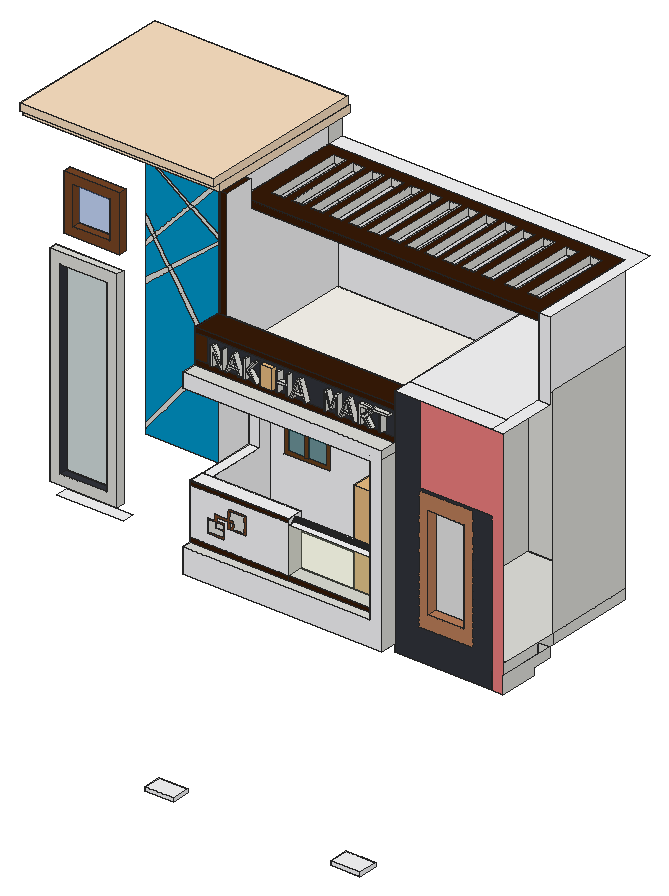
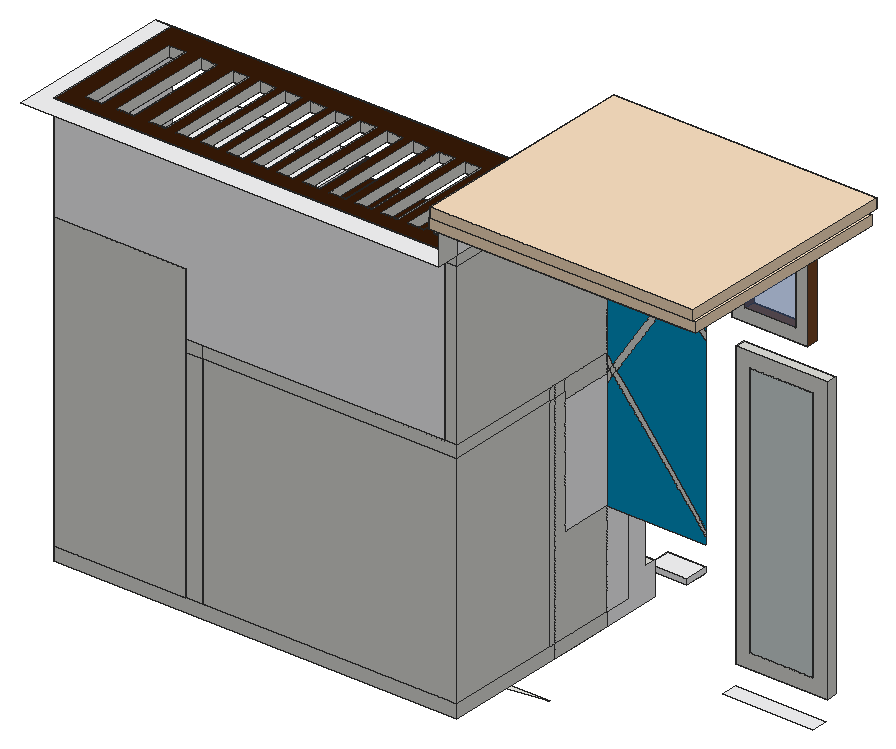
# SketchUp Ruby script. Lengths in inches.
U = 1.inch
M = Sketchup.active_model
def pt(a) = Geom::Point3d.new(a.map { |v| v * U })
def face(e, loops, mat)
  f = e.add_face(loops[0].map { |a| pt(a) })
  loops[1..].each { |l| e.add_face(l.map { |a| pt(a) }).erase! }
  f.material = f.back_material = mat if mat
  f
end
# faces: each face lists its corners as indices into pts; further lists are holes
def faces(e, pts, list, mat = nil) = list.each { |f| face(e, (f[0].is_a?(Array) ? f : [f]).map { |l| l.map { |i| pts[i] } }, mat) }
# xy, xz, yz: faces in a plane at the given z, y or x. An outline is a flat list of corners, or four numbers for a rectangle; further outlines are holes
def ring(l) = l.size == 4 ? [[l[0], l[1]], [l[2], l[1]], [l[2], l[3]], [l[0], l[3]]] : l.each_slice(2).to_a
def flat(e, list, mat, &to3) = list.each { |f| face(e, (f[0].is_a?(Array) ? f : [f]).map { |l| ring(l).map { |u, v| to3.(u, v) } }, mat) }
def xy(e, z, list, mat = nil) = flat(e, list, mat) { |x, y| [x, y, z] }
def xz(e, y, list, mat = nil) = flat(e, list, mat) { |x, z| [x, y, z] }
def yz(e, x, list, mat = nil) = flat(e, list, mat) { |y, z| [x, y, z] }
def lines(e, pts, list) = list.each { |a, b| e.add_line(pt(pts[a]), pt(pts[b])) }
# prism: a flat outline (further loops are holes) pulled along v
def prism(e, loops, v, mat = nil)
  f = face(e, loops, mat); d = Geom::Vector3d.new(v.map { |x| x * U })
  f.pushpull(f.normal.samedirection?(d) ? d.length : -d.length)
end
def box(e, o, s, mat = nil) = prism(e, [[o, [o[0] + s[0], o[1], o[2]], [o[0] + s[0], o[1] + s[1], o[2]], [o[0], o[1] + s[1], o[2]]]], [0, 0, s[2]], mat)
def at(x, y, z, deg = 0) = Geom::Transformation.translation(pt([x, y, z])) * Geom::Transformation.rotation(ORIGIN, Z_AXIS, deg.degrees)
def axes(o, x, y, z) = Geom::Transformation.new([*x, 0, *y, 0, *z, 0, *pt(o).to_a, 1])
def part(name) = M.definitions.add(name)
# library, detail: a bought-in or finely detailed component or shape, given as its bounding box
def library(name, o, s) = part(name).tap { |d| box(d.entities, o, s) }
def detail(e, o, s) = box(e.add_group.entities, o, s)
def put(e, d, t, mat = nil) = e.add_instance(d, t).tap { |i| i.material = mat if mat }
def group(e, t, mat = nil) = e.add_group.tap { |g| g.transformation = t; g.material = mat if mat }.entities
root = M.entities
M.materials.add("[0012_Bisque]").color = [255, 228, 196]
M.materials.add("[0013_LightCoral]1").color = [240, 128, 128]
M.materials.add("[0043_SaddleBrown]").color = [56, 27, 7]
M.materials.add("[0043_SaddleBrown]1").color = [79, 39, 10]
M.materials.add("[0097_DeepSkyBlue]").color = [0, 152, 204]
M.materials.add("[Asphalt New]").color = [84, 75, 77]
M.materials.add("[Blinds Vertical Pattern]").color = [250, 250, 252]
M.materials.add("[Color A08]").color = [66, 0, 0]
M.materials.add("[Formica Laminate Dark]").color = [50, 53, 60]
M.materials.add("[Formica Speckled Grey]").color = [94, 105, 111]
M.materials.add("[Sketchy Crosshatch Wavy]").color = [233, 233, 233]
M.materials.add("[Terrazzo Tile Light]").color = [255, 252, 244]
M.materials.add("[Translucent Glass Blue]").color = [78, 117, 186]
M.materials["[Translucent Glass Blue]"].alpha = 0.5
M.materials.add("[Translucent Glass Safety]").color = [227, 244, 187]
M.materials["[Translucent Glass Safety]"].alpha = 0.12
M.materials.add("[Translucent Glass Tinted]").color = [3, 87, 104]
M.materials["[Translucent Glass Tinted]"].alpha = 0.48
M.materials.add("[Wallpaper Dog Bone]").color = [213, 224, 224]
M.materials.add("[Wood Floor Parquet]").color = [104, 64, 28]
M.materials.add("[Wood Veneer 01]").color = [120, 70, 37]
M.materials.add("[Wood Veneer 02]").color = [190, 128, 91]
c1 = library("chau cay",[-24.34,-109.24,0],[56.46,62.58,79.69])
c2 = part("NAKSHA MART")
prism(c2.entities,[[[2.21,0.46,0],[2.21,19.72,0],[5.01,19.72,0],[13.81,5.77,0],[13.84,5.77,0],[13.84,19.72,0],[16.25,19.72,0],[16.25,0.46,0],[13.53,0.46,0],[4.67,14.54,0],[4.625,14.54,0],[4.625,0.46,0]]],[0,0,12])
prism(c2.entities,[[[18.64,0.46,0],[26.21,19.66,0],[29.16,19.66,0],[36.73,0.46,0],[33.61,0.46,0],[31.8,5.27,0],[23.03,5.27,0],[21.18,0.46,0]],[[23.91,7.48,0],[30.92,7.48,0],[27.4,16.65,0]]],[0,0,12])
prism(c2.entities,[[[76.07,0.46,0],[76.07,19.66,0],[79.02,19.66,0],[79.02,11.27,0],[87.14,11.27,0],[87.14,19.66,0],[90.09,19.66,0],[90.09,0.46,0],[87.14,0.46,0],[87.14,9.05,0],[79.02,9.05,0],[79.02,0.46,0]]],[0,0,12])
prism(c2.entities,[[[92.5,0.46,0],[100.07,19.66,0],[103.02,19.66,0],[110.59,0.46,0],[107.47,0.46,0],[105.66,5.27,0],[96.88,5.27,0],[95.04,0.46,0]],[[97.76,7.48,0],[104.77,7.48,0],[101.25,16.65,0]]],[0,0,12])
prism(c2.entities,[[[130.65,0.46,0],[130.65,19.66,0],[134.2,19.66,0],[138.42,7.84,0],[138.45,7.84,0],[142.59,19.66,0],[146.29,19.66,0],[146.29,0.46,0],[143.88,0.46,0],[143.88,16.9375,0],[143.85,16.9375,0],[139.53,4.52,0],[137.04,4.52,0],[132.73,16.59,0],[132.7,16.59,0],[132.7,0.46,0]]],[0,0,12])
prism(c2.entities,[[[147.89,0.46,0],[155.46,19.66,0],[158.41,19.66,0],[165.98,0.46,0],[162.86,0.46,0],[161.05,5.27,0],[152.27,5.27,0],[150.43,0.46,0]],[[153.16,7.48,0],[160.16,7.48,0],[156.64,16.65,0]]],[0,0,12])
prism(c2.entities,[[[168.93,0.46,0],[168.93,19.66,0],[174.3,19.66,0],[177.14,19.52,0],[178.95,19.11,0],[180.17,18.42,0],[181.04,17.51,0],[181.5625,16.39,0],[181.74,15.04,0],[181.49,13.2,0],[180.77,11.69,0],[179.48,10.4,0],[177.54,9.2,0],[184.17,0.46,0],[180.6,0.46,0],[174.54,8.45,0],[171.875,8.45,0],[171.875,0.46,0]],[[171.875,10.67,0],[173.43,10.67,0],[175.5625,10.93,0],[177.2,11.72,0],[177.8125,12.29,0],[178.25,12.95,0],[178.51,13.71,0],[178.59,14.55,0],[178.33,15.95,0],[178,16.46,0],[177.55,16.83,0],[176.06,17.29,0],[173.6875,17.45,0],[171.875,17.45,0]]],[0,0,12])
prism(c2.entities,[[[192.39,0.46,0],[192.39,17.45,0],[185.01,17.45,0],[185.01,19.66,0],[202.73,19.66,0],[202.73,17.45,0],[195.34,17.45,0],[195.34,0.46,0]]],[0,0,12])
xy(c2.entities,0,[[39.47,0.46,39.47,19.66,42.42,19.66,42.42,10.25,50.46,19.66,53.43,19.66,45.68,10.61,54.91,0.46,51.37,0.46,42.42,10.25,42.42,0.46]])
xy(c2.entities,12,[[39.47,0.46,42.42,0.46,42.42,10.25,51.37,0.46,54.91,0.46,45.68,10.61,53.43,19.66,50.46,19.66,42.42,10.25,42.42,19.66,39.47,19.66]])
xz(c2.entities,0.46,[[39.47,0,42.42,12],[51.37,0,54.91,12]])
xz(c2.entities,19.66,[[39.47,0,42.42,12],[50.46,0,53.43,12]])
yz(c2.entities,39.47,[[0.46,0,19.66,12]])
yz(c2.entities,42.42,[[0.46,0,10.25,12],[10.25,0,19.66,12]])
p = [[42.42,10.25,0],[51.37,0.46,0],[51.37,0.46,12],[42.42,10.25,12],[54.91,0.46,0],[45.68,10.61,0],
  [45.68,10.61,12],[54.91,0.46,12],[50.46,19.66,0],[50.46,19.66,12],[53.43,19.66,0],[53.43,19.66,12]]
faces(c2.entities,p,[[0,1,2,3],[4,5,6,7],[8,0,3,9],[5,10,11,6]])
detail(c2.entities,[57.85,0,0],[14.25,20.125,12])
xy(root,66.6875,[[328.59,26.375,349.16,29.3125],[198.03,27.5,217.83,29.3125],[198.03,29.3125,199.85,39.87],[199.85,29.3125,216.33,39.87],[216.33,29.3125,217.83,39.87],
  [328.59,29.3125,330.16,39.87],[330.16,29.3125,347.47,39.87],[347.47,29.3125,349.16,39.87]])
xy(root,69.375,[[328.59,26.375,349.16,39.87],[198.03,27.5,217.83,39.87]],"[Blinds Vertical Pattern]")
xy(root,108.13,[[239.11,191.13,244.8,194.19],[247.86,191.13,253.55,194.19],[256.61,191.13,262.3,194.19],[265.86,191.13,271.55,194.19]],"[Formica Laminate Dark]")
xy(root,124.1875,[[271.54,153.45,339.34,194.19],[339.34,153.45,347.47,180.38]],"[Formica Laminate Dark]")
xy(root,125.11,[[19.23,173.82,65.86,182.32]],"[Blinds Vertical Pattern]")
xy(root,127.39,[[239.11,191.13,244.8,194.19],[247.86,191.13,253.55,194.19],[256.61,191.13,262.3,194.19],[265.86,191.13,271.55,194.19]])
xy(root,129,[[[132.29,142.51,271.54,194.19],[133.75,159.42,143.75,170.29]],[339.34,180.38,347.47,194.19],[132.29,194.19,339.34,207.2],[132.29,207.2,339.34,270.27]])
xy(root,135.61,[[18.61,168.38,65.8,173.82]])
xy(root,136,[[132.29,159.82,139.39,210.08],[271.54,166.83,339.34,270.27],[132.29,210.08,262.84,270.27]])
xy(root,136,[[139.39,159.82,262.84,210.08]],"[Terrazzo Tile Light]")
xy(root,143.06,[[26.07,168.38,58.34,173.82]],"[Formica Laminate Dark]")
xy(root,146.0625,[[132.29,142.51,262.84,148.875]])
xy(root,149.125,[[201.12,148.875,262.84,159.82]])
xy(root,155.77,[[294.84,153.45,320.31,160.63]],"[Wood Veneer 02]")
xy(root,180.75,[[201.12,148.875,262.84,159.82]],"[Blinds Vertical Pattern]")
xy(root,184.6875,[[132.29,148.875,201.12,159.82],[132.29,159.82,139.39,200.69]])
xy(root,184.75,[[132.29,148.875,201.12,159.82],[132.29,159.82,139.39,200.69]],"[Blinds Vertical Pattern]")
xy(root,221.125,[[294.84,153.45,320.31,160.63]],"[Wood Veneer 02]")
xy(root,245.625,[[132.29,142.51,132.29,200.69,139.39,200.69,139.39,210.08,262.84,210.08,262.84,142.51]],"[Terrazzo Tile Light]")
xy(root,249,[[262.84,167.76,271.54,210.08],[132.29,200.69,139.39,210.08],[132.29,210.08,262.84,270.27],[262.84,210.08,271.54,270.27]])
xy(root,255.1875,[[132.29,142.51,271.54,153.45],[132.29,153.45,271.54,173.82],[132.29,173.82,138.29,200.69],[132.29,200.69,138.29,207.2],[132.29,207.2,138.29,210.08],
  [132.29,210.08,138.29,270.27]])
xy(root,255.1875,[[138.29,173.82,271.54,270.27]],"[Terrazzo Tile Light]")
xy(root,274.4,[[26.07,168.38,58.34,173.82]],"[Formica Laminate Dark]")
xy(root,275.125,[[132.29,153.45,271.54,173.82]])
xy(root,278.625,[[132.29,153.45,271.54,173.82]],"[0043_SaddleBrown]")
xy(root,281.86,[[18.61,168.38,65.8,173.82]])
xy(root,287.6875,[[271.54,153.45,339.34,166.83],[339.34,153.45,347.47,194.64],[271.54,166.83,339.34,270.27]],"[Blinds Vertical Pattern]")
xy(root,294.76,[[28.5625,168.13,67.5625,173.82]],"[Wood Veneer 01]")
xy(root,301.09,[[34.89,168.13,61.24,173.82]],"[Wood Veneer 01]")
xy(root,327.44,[[34.89,168.13,61.24,173.82]],"[Wood Veneer 01]")
xy(root,333.76,[[28.5625,168.13,67.5625,173.82]],"[Wood Veneer 01]")
xy(root,337.4,[[132.29,194.64,138.29,270.27]])
xy(root,337.4,[[[138.29,194.64,339.34,270.27],[142.56,207.87,151.06,261.56],[156,207.87,164.5,261.56],[169.44,207.87,177.94,261.56],[182.87,207.87,191.37,261.56],[196.31,207.87,204.81,261.56],[209.75,207.87,218.25,261.56],[223.19,207.87,231.69,261.56],[236.12,207.87,244.62,261.56],[249.06,207.87,257.56,261.56],[262,207.87,270.5,261.56],[274.94,207.87,283.44,261.56],[321.5,207.87,330,261.56],[288.87,207.87,297.37,261.56],[305.25,207.87,313.75,261.56]]],"[0043_SaddleBrown]")
xy(root,342.375,[[[132.29,194.64,339.34,270.27],[142.56,207.87,151.06,261.56],[156,207.87,164.5,261.56],[169.44,207.87,177.94,261.56],[182.87,207.87,191.37,261.56],[196.31,207.87,204.81,261.56],[209.75,207.87,218.25,261.56],[223.19,207.87,231.69,261.56],[236.12,207.87,244.62,261.56],[249.06,207.87,257.56,261.56],[262,207.87,270.5,261.56],[274.94,207.87,283.44,261.56],[288.87,207.87,297.37,261.56],[305.25,207.87,313.75,261.56],[321.5,207.87,330,261.56]]],"[0043_SaddleBrown]")
xy(root,342.375,[[339.34,194.64,347.47,194.64,347.47,281.71,132.29,281.71,132.29,270.27,339.34,270.27]],"[Blinds Vertical Pattern]")
xy(root,355.27,[[132.29,173.82,138.29,194.64]],"[0043_SaddleBrown]")
xy(root,358.25,[[5.9375,173.82,132.29,281.71],[132.29,194.64,137.48,270.27],[132.29,270.27,137.48,281.71]])
xy(root,358.25,[[0,168.63,17.38,173.82],[17.38,168.63,137.48,173.82],[0,173.82,5.9375,281.71],[132.29,173.82,137.48,194.64]],"[0012_Bisque]")
xy(root,363.3125,[[1.4375,168.63,136.67,281.71]])
xy(root,363.3125,[[1.4375,163.88,136.67,168.63],[0,168.63,1.4375,281.71],[136.67,168.63,137.48,281.71]],"[0012_Bisque]")
xy(root,368.5,[[1.4375,163.88,136.67,281.71]],"[0012_Bisque]")
xz(root,26.375,[[328.59,66.6875,349.16,69.375]],"[Blinds Vertical Pattern]")
xz(root,27.5,[[198.03,66.6875,217.83,69.375]],"[Blinds Vertical Pattern]")
xz(root,39.87,[[198.03,66.6875,217.83,69.375],[328.59,66.6875,334.94,69.375],[334.94,66.6875,339.34,69.375],[339.34,66.6875,349.16,69.375]],"[Blinds Vertical Pattern]")
xz(root,142.51,[[132.29,129,271.54,129,271.54,255.1875,132.29,255.1875,132.29,245.625,262.84,245.625,262.84,146.0625,132.29,146.0625]],"[Blinds Vertical Pattern]")
xz(root,148.875,[[145.74,157.27,155.1,157.27,155.1,160.82,149.79,160.82,149.79,164.57,145.74,164.57],[151.1,161.72,155.1,164.57],[159.85,164.57,161.67,167.94],[163.04,164.57,170.04,164.57,170.04,174.88,159.85,174.88,159.85,169.63,163.04,169.63],[132.29,184.6875,201.12,184.75]])
xz(root,148.875,[[132.29,146.0625,201.12,149.125],[201.12,146.0625,262.84,149.125],[132.29,181.99,201.12,184.6875]],"[0043_SaddleBrown]")
xz(root,148.875,[[[132.29,149.125,201.12,181.99],[144.58,156.11,144.58,165.73,149.79,165.73,149.79,169.63,158.99,169.63,158.99,176.01,171.24,176.01,171.24,163.51,158.99,163.51,158.99,167.94,151.1,167.94,151.1,165.73,156.26,165.73,156.26,156.11]]],"[Blinds Vertical Pattern]")
xz(root,148.875,[[201.12,149.125,262.84,180.75]],"[Translucent Glass Safety]")
xz(root,148.875,[[[144.58,156.11,156.26,156.11,156.26,165.73,151.1,165.73,151.1,167.94,158.99,167.94,158.99,163.51,171.24,163.51,171.24,176.01,158.99,176.01,158.99,169.63,149.79,169.63,149.79,165.73,144.58,165.73],[163.04,164.57,163.04,169.63,159.85,169.63,159.85,174.88,170.04,174.88,170.04,164.57],[145.74,157.27,145.74,164.57,149.79,164.57,149.79,160.82,155.1,160.82,155.1,161.72,151.1,161.72,151.1,164.57,155.1,164.57,155.1,157.27],[159.85,164.57,161.67,167.94]]],"[Wood Veneer 01]")
xz(root,153.45,[[339.34,124.1875,347.47,124.1875,347.47,287.6875,289.09,287.6875,289.09,233.28,339.34,233.28]],"[0013_LightCoral]1")
xz(root,153.45,[[132.29,255.1875,271.54,258.83],[132.29,275.125,271.54,278.625]],"[0043_SaddleBrown]")
xz(root,153.45,[[132.29,258.83,140.34,275.125]],"[0043_SaddleBrown]1")
xz(root,153.45,[[271.54,124.1875,339.34,124.1875,339.34,233.28,289.09,233.28,289.09,231.5,326.23,231.5,326.23,145.9375,288.92,145.9375,288.92,231.5,289.09,231.5,289.09,287.6875,271.54,287.6875],[140.34,258.83,271.54,275.125]],"[Formica Laminate Dark]")
xz(root,153.45,[[[288.92,145.9375,326.23,231.5],[294.84,155.77,320.31,221.125]]],"[Wood Veneer 02]")
xz(root,159.82,[[132.29,136,139.39,184.6875],[132.29,184.6875,139.39,184.75],[139.39,184.6875,201.12,184.75]])
xz(root,159.82,[[139.39,136,139.39,184.6875,201.12,184.6875,201.12,149.125,262.84,149.125,262.84,136]],"[Blinds Vertical Pattern]")
xz(root,159.82,[[201.12,149.125,262.84,180.75]],"[Translucent Glass Safety]")
xz(root,160.63,[[294.84,155.77,320.31,221.125]],"[Sketchy Crosshatch Wavy]")
xz(root,163.88,[[1.4375,363.3125,136.67,368.5]],"[0012_Bisque]")
xz(root,168.13,[[[28.5625,294.76,67.5625,333.76],[34.89,301.09,61.24,327.44]]],"[Wood Veneer 01]")
xz(root,168.38,[[[18.61,135.61,65.8,281.86],[26.07,143.06,58.34,274.4]]])
xz(root,168.63,[[0,358.25,137.48,363.3125]],"[0012_Bisque]")
xz(root,173.82,[[[18.61,135.61,65.8,281.86],[26.07,143.06,58.34,274.4]],[81.27,188.4,128.85,246.23,127.14,248.81,81.27,191.96],[132.29,241.04,132.29,245.625,130.55,248.28,128.85,246.23],[132.29,245.625,132.29,250.41,130.55,248.28],[128.85,246.23,130.55,248.28,128.83,250.89,127.14,248.81],
  [130.55,248.28,132.29,250.41,132.29,255.1875,128.83,250.89],[127.14,248.81,128.83,250.89,100.1,294.61,97.95,292.84],[132.29,255.1875,138.29,275.125],[132.29,275.125,133.19,278.625],[133.19,275.125,138.29,278.625],
  [132.29,278.625,133.19,355.27],[81.27,279.07,97.95,292.84,96.41,295.17,81.27,283],[97.95,292.84,100.1,294.61,98.58,296.91,96.41,295.17],[100.1,294.61,132.29,321.1875,132.29,324.01,98.58,296.91],[[28.5625,294.76,67.5625,333.76],[34.89,301.09,61.24,327.44]],
  [96.41,295.17,98.58,296.91,89.2,311.1875,87.22,309.02],[81.27,302.53,87.22,309.02,85.9,311.01,81.27,305.99],[87.22,309.02,89.2,311.1875,87.9,313.17,85.9,311.01],[85.9,311.01,87.9,313.17,81.27,323.25,81.27,317.99],[89.2,311.1875,112.875,337.04,111.05,338.27,87.9,313.17],
  [132.29,324.01,132.29,327.53,114.8,339.14,112.875,337.04],[112.875,337.04,114.8,339.14,112.97,340.36,111.05,338.27],[111.05,338.27,112.97,340.36,86.01,358.25,81.27,358.25],[114.8,339.14,132.29,358.25,129.47,358.25,112.97,340.36]])
xz(root,173.82,[[133.19,278.625,138.29,355.27]],"[0043_SaddleBrown]")
xz(root,173.82,[[132.29,184.75,132.29,241.04,128.85,246.23,81.27,188.4,81.27,184.84],[81.27,191.96,127.14,248.81,97.95,292.84,81.27,279.07],[128.83,250.89,132.29,255.1875,132.29,321.1875,100.1,294.61],[81.27,283,96.41,295.17,87.22,309.02,81.27,302.53],[98.58,296.91,132.29,324.01,112.875,337.04,89.2,311.1875],
  [81.27,305.99,85.9,311.01,81.27,317.99],[87.9,313.17,111.05,338.27,81.27,358.25,81.27,323.25],[132.29,327.53,132.29,358.25,114.8,339.14],[112.97,340.36,129.47,358.25,86.01,358.25]],"[0097_DeepSkyBlue]")
xz(root,173.82,[[138.29,255.1875,271.54,275.125],[138.29,275.125,271.54,278.625]],"[Color A08]")
xz(root,173.82,[[34.89,301.09,61.24,327.44]],"[Translucent Glass Blue]")
xz(root,173.82,[[26.07,143.06,58.34,274.4]],"[Wallpaper Dog Bone]")
xz(root,180.38,[[339.34,124.1875,347.47,129]])
xz(root,191.13,[[239.11,108.13,244.8,127.39],[247.86,108.13,253.55,127.39],[256.61,108.13,262.3,127.39],[265.86,108.13,271.55,127.39]],"[Formica Laminate Dark]")
xz(root,194.19,[[239.11,108.13,244.8,127.39],[247.86,108.13,253.55,127.39],[256.61,108.13,262.3,127.39],[265.86,108.13,265.86,127.39,271.54,127.39,271.54,124.1875,271.55,124.1875,271.55,108.13],[271.54,124.1875,271.55,127.39],
  [271.55,124.1875,287,124.1875,287,129,271.54,129,271.54,127.39,271.55,127.39],[287,124.1875,339.34,129],[339.34,129,347.47,136]])
xz(root,194.64,[[132.29,337.4,138.29,342.375],[132.29,342.375,138.29,355.27]])
xz(root,194.64,[[138.29,337.4,339.34,342.375]],"[0043_SaddleBrown]")
xz(root,194.64,[[339.34,287.6875,347.47,342.375]],"[Blinds Vertical Pattern]")
xz(root,200.69,[[132.29,184.6875,139.39,184.75],[132.29,245.625,139.39,249]])
xz(root,200.69,[[132.29,184.75,139.39,245.625]],"[Blinds Vertical Pattern]")
xz(root,207.87,[[142.56,337.4,151.06,342.375],[156,337.4,164.5,342.375],[169.44,337.4,177.94,342.375],[182.87,337.4,191.37,342.375],[196.31,337.4,204.81,342.375],
  [209.75,337.4,218.25,342.375],[223.19,337.4,231.69,342.375],[236.12,337.4,244.62,342.375],[249.06,337.4,257.56,342.375],[262,337.4,270.5,342.375],
  [274.94,337.4,283.44,342.375],[288.87,337.4,297.37,342.375],[305.25,337.4,313.75,342.375],[321.5,337.4,330,342.375]])
xz(root,210.08,[[132.29,136,139.39,249],[139.39,245.625,262.84,249]])
xz(root,210.08,[[[139.39,136,262.84,245.625],[212.31,140.93,240.81,230.93],[149.18,180.3125,181.93,229.875]]],"[Blinds Vertical Pattern]")
xz(root,210.08,[[216.73,145.34,236.4,226.52],[152.18,183.31,163.88,226.875],[166.375,183.31,178.93,226.875]],"[Translucent Glass Tinted]")
xz(root,210.08,[[[212.31,140.93,240.81,230.93],[216.73,145.34,236.4,226.52]],[[149.18,180.3125,181.93,229.875],[152.18,183.31,178.93,226.875]],[163.88,183.31,166.375,226.875]],"[Wood Floor Parquet]")
xz(root,261.56,[[142.56,337.4,151.06,342.375],[156,337.4,164.5,342.375],[169.44,337.4,177.94,342.375],[182.87,337.4,191.37,342.375],[196.31,337.4,204.81,342.375],
  [209.75,337.4,218.25,342.375],[223.19,337.4,231.69,342.375],[236.12,337.4,244.62,342.375],[249.06,337.4,257.56,342.375],[262,337.4,270.5,342.375],
  [274.94,337.4,283.44,342.375],[288.87,337.4,297.37,342.375],[305.25,337.4,313.75,342.375],[321.5,337.4,330,342.375]])
xz(root,270.27,[[132.29,129,339.34,136],[132.29,136,262.84,249],[262.84,136,271.54,249],[271.54,136,339.34,287.6875],[132.29,249,262.84,255.1875],
  [262.84,249,271.54,255.1875],[132.29,255.1875,138.29,337.4],[132.29,337.4,339.34,342.375]])
xz(root,270.27,[[138.29,255.1875,271.54,255.1875,271.54,287.6875,339.34,287.6875,339.34,337.4,138.29,337.4]],"[Blinds Vertical Pattern]")
xz(root,281.71,[[0,358.25,137.48,363.3125],[1.4375,363.3125,136.67,368.5]],"[0012_Bisque]")
yz(root,0,[[168.63,358.25,281.71,363.3125]],"[0012_Bisque]")
yz(root,1.4375,[[163.88,363.3125,281.71,368.5]],"[0012_Bisque]")
yz(root,18.61,[[168.38,135.61,173.82,281.86]])
yz(root,26.07,[[168.38,143.06,173.82,274.4]],"[Formica Laminate Dark]")
yz(root,28.5625,[[168.13,294.76,173.82,333.76]],"[Wood Veneer 01]")
yz(root,34.89,[[168.13,301.09,173.82,327.44]],"[Wood Veneer 01]")
yz(root,58.34,[[168.38,143.06,173.82,274.4]],"[Formica Laminate Dark]")
yz(root,61.24,[[168.13,301.09,173.82,327.44]],"[Wood Veneer 01]")
yz(root,65.8,[[168.38,135.61,173.82,281.86]])
yz(root,67.5625,[[168.13,294.76,173.82,333.76]],"[Wood Veneer 01]")
yz(root,132.29,[[173.82,129,207.2,136],[207.2,129,270.27,136],[173.82,136,207.2,136,207.2,249,200.69,249,200.69,184.6875,173.82,184.6875],[207.2,136,210.08,249],[210.08,136,270.27,249],
  [148.875,184.6875,159.82,184.75],[159.82,184.6875,173.82,184.75],[173.82,184.6875,200.69,184.75],[142.51,245.625,173.82,255.1875],[173.82,245.625,200.69,255.1875],
  [200.69,249,207.2,255.1875],[207.2,249,210.08,255.1875],[210.08,249,270.27,255.1875],[173.82,255.1875,173.82,355.27,194.64,355.27,194.64,337.4,270.27,337.4,270.27,255.1875],[194.64,337.4,270.27,342.375],
  [270.27,342.375,281.71,358.25]])
yz(root,132.29,[[142.51,129,142.51,146.0625,148.875,146.0625,148.875,184.6875,159.82,184.6875,159.82,136,173.82,136,173.82,129],[159.82,136,173.82,184.6875],[173.82,184.75,200.69,245.625],[194.64,342.375,270.27,358.25],[173.82,355.27,194.64,358.25]],"[Blinds Vertical Pattern]")
yz(root,132.29,[[153.45,255.1875,173.82,275.125],[153.45,275.125,173.82,278.625]],"[Color A08]")
yz(root,136.67,[[163.88,363.3125,281.71,368.5]],"[0012_Bisque]")
yz(root,137.48,[[168.63,358.25,281.71,363.3125]],"[0012_Bisque]")
yz(root,138.29,[[173.82,255.1875,270.27,255.1875,270.27,337.4,194.64,337.4,194.64,355.27,173.82,355.27]],"[Blinds Vertical Pattern]")
yz(root,139.39,[[159.82,184.6875,200.69,184.75],[200.69,245.625,210.08,249]])
yz(root,139.39,[[159.82,136,210.08,136,210.08,245.625,200.69,245.625,200.69,184.6875,159.82,184.6875]],"[Blinds Vertical Pattern]")
yz(root,142.56,[[207.87,337.4,261.56,342.375]])
yz(root,151.06,[[207.87,337.4,261.56,342.375]])
yz(root,156,[[207.87,337.4,261.56,342.375]])
yz(root,164.5,[[207.87,337.4,261.56,342.375]])
yz(root,169.44,[[207.87,337.4,261.56,342.375]])
yz(root,177.94,[[207.87,337.4,261.56,342.375]])
yz(root,182.87,[[207.87,337.4,261.56,342.375]])
yz(root,191.37,[[207.87,337.4,261.56,342.375]])
yz(root,196.31,[[207.87,337.4,261.56,342.375]])
yz(root,198.03,[[27.5,66.6875,39.87,69.375]],"[Blinds Vertical Pattern]")
yz(root,201.12,[[148.875,149.125,159.82,180.75],[154.07,181.21,153.74,181.25,153.44,181.375,153.18,181.57,152.99,181.83,152.86,182.13,152.82,182.46,152.86,182.78,152.99,183.08,153.18,183.34,153.44,183.54,153.74,183.66,154.07,183.71,154.39,183.66,154.69,183.54,154.95,183.34,155.15,183.08,155.28,182.78,155.32,182.46,155.28,182.13,155.15,181.83,154.95,181.57,154.69,181.375,154.39,181.25],[148.875,184.6875,159.82,184.75]])
yz(root,201.12,[[[148.875,180.75,159.82,184.6875],[154.07,181.21,153.74,181.25,153.44,181.375,153.18,181.57,152.99,181.83,152.86,182.13,152.82,182.46,152.86,182.78,152.99,183.08,153.18,183.34,153.44,183.54,153.74,183.66,154.07,183.71,154.39,183.66,154.69,183.54,154.95,183.34,155.15,183.08,155.28,182.78,155.32,182.46,155.28,182.13,155.15,181.83,154.95,181.57,154.69,181.375,154.39,181.25]]],"[Blinds Vertical Pattern]")
yz(root,204.81,[[207.87,337.4,261.56,342.375]])
yz(root,209.75,[[207.87,337.4,261.56,342.375]])
yz(root,217.83,[[27.5,66.6875,39.87,69.375]],"[Blinds Vertical Pattern]")
yz(root,218.25,[[207.87,337.4,261.56,342.375]])
yz(root,223.19,[[207.87,337.4,261.56,342.375]])
yz(root,231.69,[[207.87,337.4,261.56,342.375]])
yz(root,236.12,[[207.87,337.4,261.56,342.375]])
yz(root,239.11,[[191.13,108.13,194.19,127.39]],"[Formica Laminate Dark]")
yz(root,244.62,[[207.87,337.4,261.56,342.375]])
yz(root,244.8,[[191.13,108.13,194.19,127.39]],"[Formica Laminate Dark]")
yz(root,247.86,[[191.13,108.13,194.19,127.39]],"[Formica Laminate Dark]")
yz(root,249.06,[[207.87,337.4,261.56,342.375]])
yz(root,253.55,[[191.13,108.13,194.19,127.39]],"[Formica Laminate Dark]")
yz(root,256.61,[[191.13,108.13,194.19,127.39]],"[Formica Laminate Dark]")
yz(root,257.56,[[207.87,337.4,261.56,342.375]])
yz(root,262,[[207.87,337.4,261.56,342.375]])
yz(root,262.3,[[191.13,108.13,194.19,127.39]],"[Formica Laminate Dark]")
yz(root,262.84,[[210.08,136,270.27,249],[148.875,149.125,159.82,180.75],[167.76,245.625,210.08,249]])
yz(root,262.84,[[159.82,136,159.82,146.0625,167.76,146.0625,167.76,245.625,210.08,245.625,210.08,136],[[142.51,146.0625,142.51,245.625,167.76,245.625,167.76,146.0625,159.82,146.0625,159.82,180.75,148.875,180.75,148.875,146.0625],[154.07,181.21,154.39,181.25,154.69,181.375,154.95,181.57,155.15,181.83,155.28,182.13,155.32,182.46,155.28,182.78,155.15,183.08,154.95,183.34,154.69,183.54,154.39,183.66,154.07,183.71,153.74,183.66,153.44,183.54,153.18,183.34,152.99,183.08,152.86,182.78,152.82,182.46,152.86,182.13,152.99,181.83,153.18,181.57,153.44,181.375,153.74,181.25]]],"[Blinds Vertical Pattern]")
yz(root,265.86,[[191.13,108.13,194.19,127.39]],"[Formica Laminate Dark]")
yz(root,270.5,[[207.87,337.4,261.56,342.375]])
yz(root,271.54,[[153.45,124.1875,194.19,129],[142.51,129,153.45,249],[166.83,136,270.27,136,270.27,249,167.76,249,167.76,255.1875,166.83,255.1875],[142.51,249,153.45,255.1875],[167.76,249,210.08,255.1875],
  [210.08,249,270.27,255.1875],[153.45,255.1875,166.83,275.125],[166.83,255.1875,167.76,275.125],[167.76,255.1875,173.82,275.125],[153.45,275.125,166.83,278.625],
  [166.83,275.125,167.76,278.625],[167.76,275.125,173.82,278.625]])
yz(root,271.54,[[153.45,278.625,166.83,287.6875]],"[Asphalt New]")
yz(root,271.54,[[173.82,255.1875,173.82,278.625,166.83,278.625,166.83,287.6875,210.08,287.6875,210.08,255.1875],[210.08,255.1875,270.27,287.6875]],"[Blinds Vertical Pattern]")
yz(root,271.55,[[191.13,108.13,194.19,127.39]],"[Formica Laminate Dark]")
yz(root,274.94,[[207.87,337.4,261.56,342.375]])
yz(root,283.44,[[207.87,337.4,261.56,342.375]])
yz(root,288.87,[[207.87,337.4,261.56,342.375]])
yz(root,294.84,[[153.45,155.77,160.63,221.125]],"[Wood Veneer 02]")
yz(root,297.37,[[207.87,337.4,261.56,342.375]])
yz(root,305.25,[[207.87,337.4,261.56,342.375]])
yz(root,313.75,[[207.87,337.4,261.56,342.375]])
yz(root,320.31,[[153.45,155.77,160.63,221.125]],"[Wood Veneer 02]")
yz(root,321.5,[[207.87,337.4,261.56,342.375]])
yz(root,328.59,[[26.375,66.6875,39.87,69.375]],"[Blinds Vertical Pattern]")
yz(root,330,[[207.87,337.4,261.56,342.375]])
yz(root,339.34,[[153.45,124.1875,180.38,124.1875,180.38,129,194.19,129,194.19,136,153.45,136],[180.38,124.1875,194.19,129],[194.19,129,207.2,136],[207.2,129,270.27,136],[207.2,136,270.27,287.6875],
  [194.64,337.4,270.27,342.375]])
yz(root,339.34,[[194.64,287.6875,270.27,337.4]],"[Blinds Vertical Pattern]")
yz(root,347.47,[[153.45,124.1875,180.38,124.1875,180.38,129,194.19,129,194.19,136,153.45,136]])
yz(root,349.16,[[26.375,66.6875,39.87,69.375]],"[Blinds Vertical Pattern]")
p = [[145.06,194.19,99.57],[158.57,207.2,106.65],[218.13,207.2,106.65],[197.47,194.19,99.57],[201.12,153.44,181.375],[201.12,153.74,181.25],
  [262.84,153.74,181.25],[262.84,153.44,181.375],[201.12,154.07,181.21],[262.84,154.07,181.21],[201.12,154.39,181.25],[262.84,154.39,181.25],
  [201.12,154.69,181.375],[262.84,154.69,181.375],[201.12,153.18,181.57],[262.84,153.18,181.57],[201.12,154.95,181.57],[262.84,154.95,181.57],
  [201.12,152.99,181.83],[262.84,152.99,181.83],[201.12,155.15,181.83],[262.84,155.15,181.83],[201.12,152.86,182.13],[262.84,152.86,182.13],
  [201.12,155.28,182.13],[262.84,155.28,182.13],[201.12,152.82,182.46],[262.84,152.82,182.46],[201.12,155.32,182.46],[262.84,155.32,182.46],
  [201.12,152.86,182.78],[262.84,152.86,182.78],[201.12,155.28,182.78],[262.84,155.28,182.78],[201.12,152.99,183.08],[262.84,152.99,183.08],
  [201.12,155.15,183.08],[262.84,155.15,183.08],[201.12,153.18,183.34],[262.84,153.18,183.34],[201.12,154.95,183.34],[262.84,154.95,183.34],
  [201.12,153.44,183.54],[262.84,153.44,183.54],[201.12,154.69,183.54],[262.84,154.69,183.54],[201.12,153.74,183.66],[262.84,153.74,183.66],
  [201.12,154.39,183.66],[262.84,154.39,183.66],[201.12,154.07,183.71],[262.84,154.07,183.71],[262.84,159.82,136],[262.84,153.45,136],
  [262.84,167.76,249],[262.84,142.51,249]]
faces(root,p,[[0,1,2,3]])
faces(root,p,[[4,5,6,7],[5,8,9,6],[8,10,11,9],[10,12,13,11],[14,4,7,15],[12,16,17,13],[18,14,15,19],[16,20,21,17],
  [22,18,19,23],[20,24,25,21],[26,22,23,27],[24,28,29,25],[30,26,27,31],[28,32,33,29],[34,30,31,35],[32,36,37,33],
  [38,34,35,39],[36,40,41,37],[42,38,39,43],[40,44,45,41],[46,42,43,47],[44,48,49,45],[50,46,47,51],[48,50,51,49]],"[Formica Speckled Grey]")
lines(root,p,[[52,53],[54,55]])
put(root,c1,axes([253.08,247.41,136],[0.6162,0,0],[0,0.8,0],[0,0,0.98]))
put(root,c2,axes([144.33,153.45,260.2],[0.61916,0,0],[0,0,0.68],[0,-0.3,0]))
